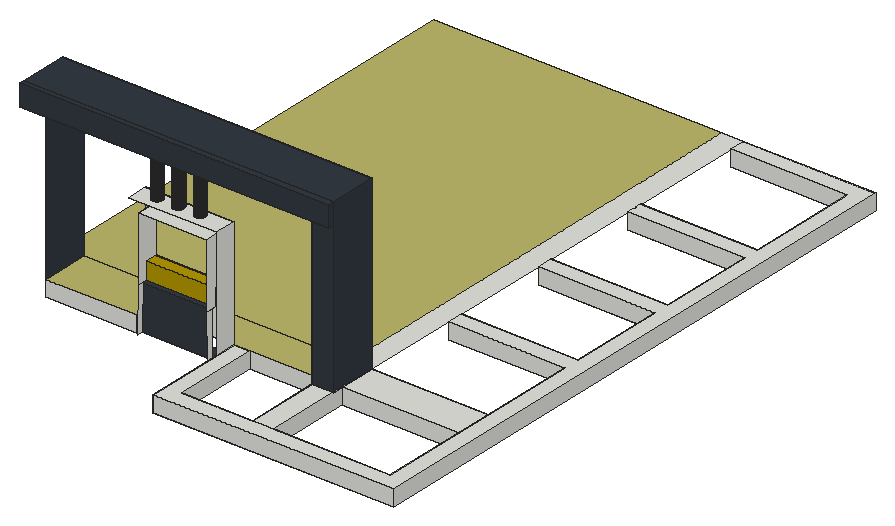
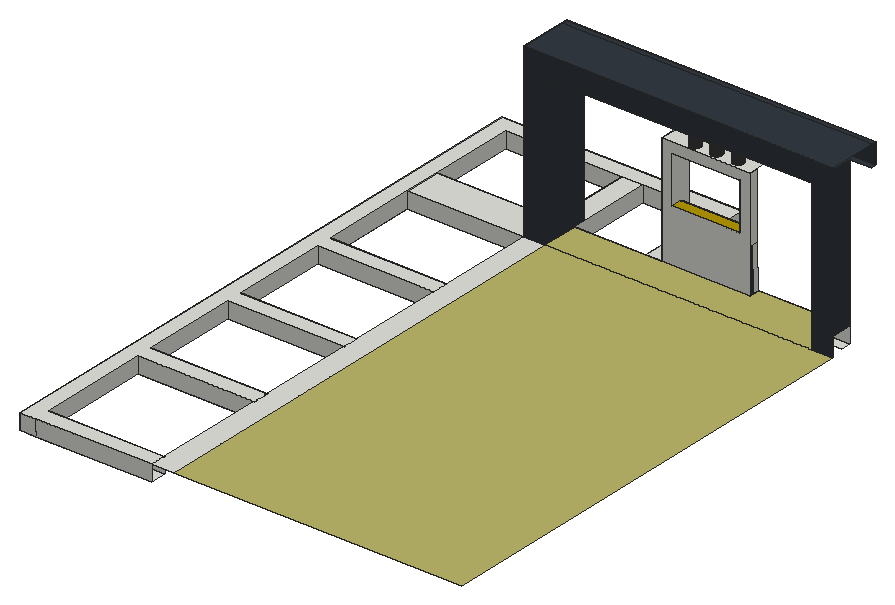
# SketchUp Ruby script. Lengths in inches.
U = 1.inch
M = Sketchup.active_model
def pt(a) = Geom::Point3d.new(a.map { |v| v * U })
def face(e, loops, mat)
  f = e.add_face(loops[0].map { |a| pt(a) })
  loops[1..].each { |l| e.add_face(l.map { |a| pt(a) }).erase! }
  f.material = f.back_material = mat if mat
  f
end
# faces: each face lists its corners as indices into pts; further lists are holes
def faces(e, pts, list, mat = nil) = list.each { |f| face(e, (f[0].is_a?(Array) ? f : [f]).map { |l| l.map { |i| pts[i] } }, mat) }
# xy, xz, yz: faces in a plane at the given z, y or x. An outline is a flat list of corners, or four numbers for a rectangle; further outlines are holes
def ring(l) = l.size == 4 ? [[l[0], l[1]], [l[2], l[1]], [l[2], l[3]], [l[0], l[3]]] : l.each_slice(2).to_a
def flat(e, list, mat, &to3) = list.each { |f| face(e, (f[0].is_a?(Array) ? f : [f]).map { |l| ring(l).map { |u, v| to3.(u, v) } }, mat) }
def xy(e, z, list, mat = nil) = flat(e, list, mat) { |x, y| [x, y, z] }
def xz(e, y, list, mat = nil) = flat(e, list, mat) { |x, z| [x, y, z] }
def yz(e, x, list, mat = nil) = flat(e, list, mat) { |y, z| [x, y, z] }
def lines(e, pts, list) = list.each { |a, b| e.add_line(pt(pts[a]), pt(pts[b])) }
# prism: a flat outline (further loops are holes) pulled along v
def prism(e, loops, v, mat = nil)
  f = face(e, loops, mat); d = Geom::Vector3d.new(v.map { |x| x * U })
  f.pushpull(f.normal.samedirection?(d) ? d.length : -d.length)
end
def box(e, o, s, mat = nil) = prism(e, [[o, [o[0] + s[0], o[1], o[2]], [o[0] + s[0], o[1] + s[1], o[2]], [o[0], o[1] + s[1], o[2]]]], [0, 0, s[2]], mat)
def at(x, y, z, deg = 0) = Geom::Transformation.translation(pt([x, y, z])) * Geom::Transformation.rotation(ORIGIN, Z_AXIS, deg.degrees)
def axes(o, x, y, z) = Geom::Transformation.new([*x, 0, *y, 0, *z, 0, *pt(o).to_a, 1])
def part(name) = M.definitions.add(name)
# library, detail: a bought-in or finely detailed component or shape, given as its bounding box
def library(name, o, s) = part(name).tap { |d| box(d.entities, o, s) }
def detail(e, o, s) = box(e.add_group.entities, o, s)
def put(e, d, t, mat = nil) = e.add_instance(d, t).tap { |i| i.material = mat if mat }
def group(e, t, mat = nil) = e.add_group.tap { |g| g.transformation = t; g.material = mat if mat }.entities
root = M.entities
M.materials.add("[0046_Gold]").color = [178, 150, 0]
M.materials.add("[0057_DarkKhaki]").color = [188, 182, 106]
M.materials.add("[0111_SlateGray]").color = [51, 58, 66]
xy(root,810,[[388.78,0,388.78,114,406.78,114,406.78,18,486,18,486,114,510,114,510,18,641,18,641,264,510,264,510,282,641,282,641,390,510,390,510,408,641,408,641,516,510,516,510,534,641,534,641,678,659,678,659,0],[186,102,288.84,114],[510,114,641,156],[510,660,641,678]])
xy(root,817.66,[[299.18,96,378.44,114]],"[0111_SlateGray]")
xy(root,828,[[388.78,0,659,0,659,678,510,678,510,660,641,660,641,534,510,534,510,516,641,516,641,408,510,408,510,390,641,390,641,282,510,282,510,264,641,264,641,18,406.78,18,406.78,114,388.78,114],[486,18,510,102],[486,102,510,114],[486,114,510,156],[510,114,641,156],
  [486,156,510,678]])
xy(root,828,[[186,102,288.84,102,288.84,114,486,114,486,156,186,156],[162,156,486,678]],"[0057_DarkKhaki]")
xy(root,867.66,[[300.19,96,377.43,101]],"[0111_SlateGray]")
xy(root,887.35,[[300.19,101,377.43,114]],"[0046_Gold]")
xy(root,940.57,[[300.19,90,377.43,114]])
xy(root,951.92,[[[288.84,90,388.78,114],[309.5,98.9375,308.875,98.96,308.25,99.05,307.64,99.21,307.05,99.43,306.49,99.71,305.96,100.04,305.47,100.43,305.02,100.87,304.62,101.35,304.27,101.875,303.98,102.43,303.74,103.01,303.58,103.62,303.47,104.24,303.43,104.87,303.45,105.49,303.55,106.11,303.7,106.72,303.92,107.3125,304.2,107.875,304.53,108.41,304.92,108.9,305.36,109.35,305.84,109.75,306.37,110.1,306.92,110.39,307.51,110.62,308.11,110.79,308.73,110.9,309.36,110.9375,309.98,110.91,310.61,110.82,311.21,110.67,311.8,110.45,312.37,110.17,312.9,109.83,313.39,109.44,313.84,109.01,314.24,108.52,314.59,108,314.88,107.44,315.11,106.86,315.28,106.26,315.39,105.64,315.43,105.01,315.4,104.38,315.3125,103.76,315.16,103.15,314.9375,102.5625,314.66,102,314.32,101.47,313.94,100.98,313.5,100.53,313.01,100.125,312.49,99.78,311.93,99.49,311.35,99.25,310.75,99.08,310.13,98.98],[333.5,99.0625,332.875,99.09,332.25,99.18,331.64,99.33,331.05,99.55,330.49,99.83,329.96,100.17,329.47,100.56,329.02,100.99,328.62,101.48,328.27,102,327.98,102.56,327.74,103.14,327.58,103.74,327.47,104.36,327.43,104.99,327.45,105.62,327.55,106.24,327.7,106.85,327.92,107.4375,328.2,108,328.53,108.53,328.92,109.02,329.36,109.47,329.84,109.875,330.37,110.22,330.92,110.51,331.51,110.75,332.11,110.92,332.73,111.02,333.36,111.0625,333.98,111.04,334.61,110.95,335.21,110.79,335.8,110.57,336.37,110.29,336.9,109.96,337.39,109.57,337.84,109.13,338.24,108.65,338.59,108.125,338.88,107.57,339.11,106.99,339.28,106.38,339.39,105.76,339.43,105.13,339.4,104.51,339.3125,103.89,339.16,103.28,338.9375,102.6875,338.66,102.125,338.32,101.59,337.94,101.1,337.5,100.65,337.01,100.25,336.49,99.9,335.93,99.61,335.35,99.38,334.75,99.21,334.13,99.1],[357.5,99.625,356.875,99.65,356.25,99.74,355.64,99.9,355.05,100.11,354.49,100.39,353.96,100.73,353.47,101.12,353.02,101.56,352.62,102.04,352.27,102.5625,351.98,103.12,351.74,103.7,351.58,104.31,351.47,104.93,351.43,105.55,351.45,106.18,351.55,106.8,351.7,107.41,351.92,108,352.2,108.5625,352.53,109.09,352.92,109.59,353.36,110.04,353.84,110.4375,354.37,110.78,354.92,111.08,355.51,111.31,356.11,111.48,356.73,111.58,357.36,111.625,357.98,111.6,358.61,111.51,359.21,111.35,359.8,111.14,360.37,110.86,360.9,110.52,361.39,110.13,361.84,109.69,362.24,109.21,362.59,108.6875,362.88,108.13,363.11,107.55,363.28,106.94,363.39,106.32,363.43,105.7,363.4,105.07,363.3125,104.45,363.16,103.84,362.9375,103.25,362.66,102.6875,362.32,102.16,361.94,101.66,361.5,101.21,361.01,100.8125,360.49,100.47,359.93,100.17,359.35,99.94,358.75,99.77,358.13,99.67]],[309.5,98.9375,308.875,98.96,308.25,99.05,307.64,99.21,307.05,99.43,306.49,99.71,305.96,100.04,305.47,100.43,305.02,100.87,304.62,101.35,304.27,101.875,303.98,102.43,303.74,103.01,303.58,103.62,303.47,104.24,303.43,104.87,303.45,105.49,303.55,106.11,303.7,106.72,303.92,107.3125,304.2,107.875,304.53,108.41,304.92,108.9,305.36,109.35,305.84,109.75,306.37,110.1,306.92,110.39,307.51,110.62,308.11,110.79,308.73,110.9,309.36,110.9375,309.98,110.91,310.61,110.82,311.21,110.67,311.8,110.45,312.37,110.17,312.9,109.83,313.39,109.44,313.84,109.01,314.24,108.52,314.59,108,314.88,107.44,315.11,106.86,315.28,106.26,315.39,105.64,315.43,105.01,315.4,104.38,315.3125,103.76,315.16,103.15,314.9375,102.5625,314.66,102,314.32,101.47,313.94,100.98,313.5,100.53,313.01,100.125,312.49,99.78,311.93,99.49,311.35,99.25,310.75,99.08,310.13,98.98],[333.5,99.0625,332.875,99.09,332.25,99.18,331.64,99.33,331.05,99.55,330.49,99.83,329.96,100.17,329.47,100.56,329.02,100.99,328.62,101.48,328.27,102,327.98,102.56,327.74,103.14,327.58,103.74,327.47,104.36,327.43,104.99,327.45,105.62,327.55,106.24,327.7,106.85,327.92,107.4375,328.2,108,328.53,108.53,328.92,109.02,329.36,109.47,329.84,109.875,330.37,110.22,330.92,110.51,331.51,110.75,332.11,110.92,332.73,111.02,333.36,111.0625,333.98,111.04,334.61,110.95,335.21,110.79,335.8,110.57,336.37,110.29,336.9,109.96,337.39,109.57,337.84,109.13,338.24,108.65,338.59,108.125,338.88,107.57,339.11,106.99,339.28,106.38,339.39,105.76,339.43,105.13,339.4,104.51,339.3125,103.89,339.16,103.28,338.9375,102.6875,338.66,102.125,338.32,101.59,337.94,101.1,337.5,100.65,337.01,100.25,336.49,99.9,335.93,99.61,335.35,99.38,334.75,99.21,334.13,99.1],[357.5,99.625,356.875,99.65,356.25,99.74,355.64,99.9,355.05,100.11,354.49,100.39,353.96,100.73,353.47,101.12,353.02,101.56,352.62,102.04,352.27,102.5625,351.98,103.12,351.74,103.7,351.58,104.31,351.47,104.93,351.43,105.55,351.45,106.18,351.55,106.8,351.7,107.41,351.92,108,352.2,108.5625,352.53,109.09,352.92,109.59,353.36,110.04,353.84,110.4375,354.37,110.78,354.92,111.08,355.51,111.31,356.11,111.48,356.73,111.58,357.36,111.625,357.98,111.6,358.61,111.51,359.21,111.35,359.8,111.14,360.37,110.86,360.9,110.52,361.39,110.13,361.84,109.69,362.24,109.21,362.59,108.6875,362.88,108.13,363.11,107.55,363.28,106.94,363.39,106.32,363.43,105.7,363.4,105.07,363.3125,104.45,363.16,103.84,362.9375,103.25,362.66,102.6875,362.32,102.16,361.94,101.66,361.5,101.21,361.01,100.8125,360.49,100.47,359.93,100.17,359.35,99.94,358.75,99.77,358.13,99.67]])
xy(root,996,[[309.5,98.9375,310.13,98.98,310.75,99.08,311.35,99.25,311.93,99.49,312.49,99.78,313.01,100.125,313.5,100.53,313.94,100.98,314.32,101.47,314.66,102,304.2,102,304.27,101.875,304.62,101.35,305.02,100.87,305.47,100.43,305.96,100.04,306.49,99.71,307.05,99.43,307.64,99.21,308.25,99.05,308.875,98.96],[333.5,99.0625,334.13,99.1,334.75,99.21,335.35,99.38,335.93,99.61,336.49,99.9,337.01,100.25,337.5,100.65,337.94,101.1,338.32,101.59,338.58,102,328.27,102,328.62,101.48,329.02,100.99,329.47,100.56,329.96,100.17,330.49,99.83,331.05,99.55,331.64,99.33,332.25,99.18,332.875,99.09],[357.5,99.625,358.13,99.67,358.75,99.77,359.35,99.94,359.93,100.17,360.49,100.47,361.01,100.8125,361.5,101.21,361.94,101.66,362.2,102,352.65,102,353.02,101.56,353.47,101.12,353.96,100.73,354.49,100.39,355.05,100.11,355.64,99.9,356.25,99.74,356.875,99.65],[304.2,102,314.66,102,314.9375,102.5625,315.16,103.15,315.3125,103.76,315.4,104.38,315.43,105.01,315.39,105.64,315.28,106.26,315.11,106.86,314.88,107.44,314.59,108,314.24,108.52,313.84,109.01,313.39,109.44,312.9,109.83,312.37,110.17,311.8,110.45,311.21,110.67,310.61,110.82,309.98,110.91,309.36,110.9375,308.73,110.9,308.11,110.79,307.51,110.62,306.92,110.39,306.37,110.1,305.84,109.75,305.36,109.35,304.92,108.9,304.53,108.41,304.2,107.875,303.92,107.3125,303.7,106.72,303.55,106.11,303.45,105.49,303.43,104.87,303.47,104.24,303.58,103.62,303.74,103.01,303.98,102.43],[328.27,102,338.58,102,338.66,102.125,338.9375,102.6875,339.16,103.28,339.3125,103.89,339.4,104.51,339.43,105.13,339.39,105.76,339.28,106.38,339.11,106.99,338.88,107.57,338.59,108.125,338.24,108.65,337.84,109.13,337.39,109.57,336.9,109.96,336.37,110.29,335.8,110.57,335.21,110.79,334.61,110.95,333.98,111.04,333.36,111.0625,332.73,111.02,332.11,110.92,331.51,110.75,330.92,110.51,330.37,110.22,329.84,109.875,329.36,109.47,328.92,109.02,328.53,108.53,328.2,108,327.92,107.4375,327.7,106.85,327.55,106.24,327.45,105.62,327.43,104.99,327.47,104.36,327.58,103.74,327.74,103.14,327.98,102.56],
  [352.65,102,362.2,102,362.32,102.16,362.66,102.6875,362.9375,103.25,363.16,103.84,363.3125,104.45,363.4,105.07,363.43,105.7,363.39,106.32,363.28,106.94,363.11,107.55,362.88,108.13,362.59,108.6875,362.24,109.21,361.84,109.69,361.39,110.13,360.9,110.52,360.37,110.86,359.8,111.14,359.21,111.35,358.61,111.51,357.98,111.6,357.36,111.625,356.73,111.58,356.11,111.48,355.51,111.31,354.92,111.08,354.37,110.78,353.84,110.4375,353.36,110.04,352.92,109.59,352.53,109.09,352.2,108.5625,351.92,108,351.7,107.41,351.55,106.8,351.45,106.18,351.43,105.55,351.47,104.93,351.58,104.31,351.74,103.7,351.98,103.12,352.27,102.5625,352.62,102.04],[239.33,115.14,238.07,115.2,236.83,115.39,235.61,115.71,234.4375,116.15,233.32,116.71,232.26,117.39,231.28,118.17,230.38,119.06,229.59,120.03,228.9,121.08,228.32,122.19,227.86,123.36,227.53,124.57,227.32,125.8125,227.25,127.07,227.31,128.32,227.5,129.5625,227.8125,130.78,228.26,131.95,228.82,133.08,229.5,134.13,230.28,135.12,231.16,136.01,232.13,136.81,233.18,137.5,234.3,138.07,235.47,138.53,236.68,138.87,237.92,139.07,239.17,139.14,240.43,139.09,241.67,138.9,242.88,138.58,244.06,138.14,245.18,137.57,246.24,136.9,247.22,136.11,248.11,135.23,248.91,134.26,249.6,133.21,250.18,132.09,250.64,130.93,250.97,129.71,251.17,128.47,251.25,127.22,251.19,125.97,251,124.72,250.69,123.51,250.24,122.33,249.68,121.21,249,120.15,248.22,119.17,247.34,118.28,246.36,117.48,245.32,116.79,244.2,116.21,243.03,115.76,241.82,115.42,240.58,115.22],[442.51,115.14,441.26,115.2,440.02,115.39,438.8,115.71,437.625,116.15,436.5,116.71,435.45,117.39,434.46,118.17,433.57,119.06,432.77,120.03,432.08,121.08,431.51,122.19,431.05,123.36,430.72,124.57,430.51,125.8125,430.4375,127.07,430.49,128.32,430.68,129.5625,431,130.78,431.44,131.95,432.01,133.08,432.68,134.13,433.47,135.12,434.35,136.01,435.32,136.81,436.37,137.5,437.49,138.07,438.65,138.53,439.87,138.87,441.11,139.07,442.36,139.14,443.61,139.09,444.86,138.9,446.07,138.58,447.25,138.14,448.37,137.57,449.43,136.9,450.41,136.11,451.3,135.23,452.1,134.26,452.79,133.21,453.37,132.09,453.83,130.93,454.16,129.71,454.36,128.47,454.4375,127.22,454.38,125.97,454.19,124.72,453.87,123.51,453.43,122.33,452.87,121.21,452.19,120.15,451.41,119.17,450.52,118.28,449.55,117.48,448.5,116.79,447.39,116.21,446.22,115.76,445.01,115.42,443.77,115.22]])
xy(root,996,[[[162,96,162,102,186,102,186,156,486,156,486,102,510,102,510,96],[442.51,115.14,443.77,115.22,445.01,115.42,446.22,115.76,447.39,116.21,448.5,116.79,449.55,117.48,450.52,118.28,451.41,119.17,452.19,120.15,452.87,121.21,453.43,122.33,453.87,123.51,454.19,124.72,454.38,125.97,454.4375,127.22,454.36,128.47,454.16,129.71,453.83,130.93,453.37,132.09,452.79,133.21,452.1,134.26,451.3,135.23,450.41,136.11,449.43,136.9,448.37,137.57,447.25,138.14,446.07,138.58,444.86,138.9,443.61,139.09,442.36,139.14,441.11,139.07,439.87,138.87,438.65,138.53,437.49,138.07,436.37,137.5,435.32,136.81,434.35,136.01,433.47,135.12,432.68,134.13,432.01,133.08,431.44,131.95,431,130.78,430.68,129.5625,430.49,128.32,430.4375,127.07,430.51,125.8125,430.72,124.57,431.05,123.36,431.51,122.19,432.08,121.08,432.77,120.03,433.57,119.06,434.46,118.17,435.45,117.39,436.5,116.71,437.625,116.15,438.8,115.71,440.02,115.39,441.26,115.2],[239.33,115.14,240.58,115.22,241.82,115.42,243.03,115.76,244.2,116.21,245.32,116.79,246.36,117.48,247.34,118.28,248.22,119.17,249,120.15,249.68,121.21,250.24,122.33,250.69,123.51,251,124.72,251.19,125.97,251.25,127.22,251.17,128.47,250.97,129.71,250.64,130.93,250.18,132.09,249.6,133.21,248.91,134.26,248.11,135.23,247.22,136.11,246.24,136.9,245.18,137.57,244.06,138.14,242.88,138.58,241.67,138.9,240.43,139.09,239.17,139.14,237.92,139.07,236.68,138.87,235.47,138.53,234.3,138.07,233.18,137.5,232.13,136.81,231.16,136.01,230.28,135.12,229.5,134.13,228.82,133.08,228.26,131.95,227.8125,130.78,227.5,129.5625,227.31,128.32,227.25,127.07,227.32,125.8125,227.53,124.57,227.86,123.36,228.32,122.19,228.9,121.08,229.59,120.03,230.38,119.06,231.28,118.17,232.26,117.39,233.32,116.71,234.4375,116.15,235.61,115.71,236.83,115.39,238.07,115.2],[357.5,99.625,358.13,99.67,358.75,99.77,359.35,99.94,359.93,100.17,360.49,100.47,361.01,100.8125,361.5,101.21,361.94,101.66,362.2,102,362.32,102.16,362.66,102.6875,362.9375,103.25,363.16,103.84,363.3125,104.45,363.4,105.07,363.43,105.7,363.39,106.32,363.28,106.94,363.11,107.55,362.88,108.13,362.59,108.6875,362.24,109.21,361.84,109.69,361.39,110.13,360.9,110.52,360.37,110.86,359.8,111.14,359.21,111.35,358.61,111.51,357.98,111.6,357.36,111.625,356.73,111.58,356.11,111.48,355.51,111.31,354.92,111.08,354.37,110.78,353.84,110.4375,353.36,110.04,352.92,109.59,352.53,109.09,352.2,108.5625,351.92,108,351.7,107.41,351.55,106.8,351.45,106.18,351.43,105.55,351.47,104.93,351.58,104.31,351.74,103.7,351.98,103.12,352.27,102.5625,352.62,102.04,352.65,102,353.02,101.56,353.47,101.12,353.96,100.73,354.49,100.39,355.05,100.11,355.64,99.9,356.25,99.74,356.875,99.65],[333.5,99.0625,334.13,99.1,334.75,99.21,335.35,99.38,335.93,99.61,336.49,99.9,337.01,100.25,337.5,100.65,337.94,101.1,338.32,101.59,338.58,102,338.66,102.125,338.9375,102.6875,339.16,103.28,339.3125,103.89,339.4,104.51,339.43,105.13,339.39,105.76,339.28,106.38,339.11,106.99,338.88,107.57,338.59,108.125,338.24,108.65,337.84,109.13,337.39,109.57,336.9,109.96,336.37,110.29,335.8,110.57,335.21,110.79,334.61,110.95,333.98,111.04,333.36,111.0625,332.73,111.02,332.11,110.92,331.51,110.75,330.92,110.51,330.37,110.22,329.84,109.875,329.36,109.47,328.92,109.02,328.53,108.53,328.2,108,327.92,107.4375,327.7,106.85,327.55,106.24,327.45,105.62,327.43,104.99,327.47,104.36,327.58,103.74,327.74,103.14,327.98,102.56,328.27,102,328.62,101.48,329.02,100.99,329.47,100.56,329.96,100.17,330.49,99.83,331.05,99.55,331.64,99.33,332.25,99.18,332.875,99.09],[309.5,98.9375,310.13,98.98,310.75,99.08,311.35,99.25,311.93,99.49,312.49,99.78,313.01,100.125,313.5,100.53,313.94,100.98,314.32,101.47,314.66,102,314.9375,102.5625,315.16,103.15,315.3125,103.76,315.4,104.38,315.43,105.01,315.39,105.64,315.28,106.26,315.11,106.86,314.88,107.44,314.59,108,314.24,108.52,313.84,109.01,313.39,109.44,312.9,109.83,312.37,110.17,311.8,110.45,311.21,110.67,310.61,110.82,309.98,110.91,309.36,110.9375,308.73,110.9,308.11,110.79,307.51,110.62,306.92,110.39,306.37,110.1,305.84,109.75,305.36,109.35,304.92,108.9,304.53,108.41,304.2,107.875,303.92,107.3125,303.7,106.72,303.55,106.11,303.45,105.49,303.43,104.87,303.47,104.24,303.58,103.62,303.74,103.01,303.98,102.43,304.2,102,304.27,101.875,304.62,101.35,305.02,100.87,305.47,100.43,305.96,100.04,306.49,99.71,307.05,99.43,307.64,99.21,308.25,99.05,308.875,98.96]]],"[0111_SlateGray]")
xy(root,1020,[[162,96,510,102],[162,102,510,156]],"[0111_SlateGray]")
xz(root,0,[[388.78,810,659,828]])
xz(root,18,[[406.78,810,486,828],[510,810,641,828]])
xz(root,96,[[299.18,817.66,378.44,817.66,377.43,867.66,300.19,867.66],[162,996,510,1020]],"[0111_SlateGray]")
xz(root,101,[[300.19,867.66,377.43,887.35]],"[0046_Gold]")
xz(root,102,[[186,810,288.84,828]])
xz(root,102,[[486,828,510,996]],"[0111_SlateGray]")
xz(root,114,[[388.78,810,406.78,828],[406.78,810,486,828],[486,810,510,828],[510,810,641,828],[[288.84,828,388.78,951.92],[300.19,887.35,377.43,940.57]]])
xz(root,156,[[510,810,641,828]])
xz(root,156,[[162,828,162,1020,510,1020,510,828,486,828,486,996,186,996,186,828]],"[0111_SlateGray]")
xz(root,264,[[510,810,641,828]])
xz(root,282,[[510,810,641,828]])
xz(root,390,[[510,810,641,828]])
xz(root,408,[[510,810,641,828]])
xz(root,516,[[510,810,641,828]])
xz(root,534,[[510,810,641,828]])
xz(root,660,[[510,810,641,828]])
xz(root,678,[[510,810,641,828],[641,810,659,828]])
yz(root,186,[[102,828,156,996]],"[0111_SlateGray]")
yz(root,288.84,[[102,810,114,828]])
yz(root,300.19,[[90,867.66,101,867.66,101,887.35,114,887.35,114,940.57,90,940.57]])
yz(root,377.43,[[90,867.66,90,940.57,114,940.57,114,887.35,101,887.35,101,867.66]])
yz(root,388.78,[[0,810,90,828],[90,810,114,828],[90,828,114,951.92]])
yz(root,406.78,[[18,810,114,828]])
yz(root,486,[[18,810,114,828]])
yz(root,486,[[102,828,156,996]],"[0111_SlateGray]")
yz(root,510,[[18,810,114,828],[114,810,156,828]])
yz(root,510,[[102,828,156,1020],[96,996,102,1020]],"[0111_SlateGray]")
yz(root,641,[[18,810,114,828],[114,810,156,828],[156,810,264,828],[282,810,390,828],[408,810,516,828],
  [534,810,660,828]])
yz(root,659,[[0,810,678,828]])
p = [[300.19,90,867.66],[299.18,90,817.66],[299.18,96,817.66],[300.19,96,867.66],[378.44,90,817.66],[377.43,90,867.66],
  [377.43,96,867.66],[378.44,96,817.66],[308.875,98.96,951.92],[309.5,98.9375,951.92],[309.5,98.9375,996],[308.875,98.96,996],
  [310.13,98.98,951.92],[310.13,98.98,996],[308.25,99.05,951.92],[308.25,99.05,996],[310.75,99.08,951.92],[310.75,99.08,996],
  [307.64,99.21,951.92],[307.64,99.21,996],[311.35,99.25,951.92],[311.35,99.25,996],[332.25,99.18,951.92],[332.875,99.09,951.92],
  [332.875,99.09,996],[332.25,99.18,996],[333.5,99.0625,951.92],[333.5,99.0625,996],[334.13,99.1,951.92],[334.13,99.1,996],
  [334.75,99.21,951.92],[334.75,99.21,996],[307.05,99.43,951.92],[307.05,99.43,996],[331.64,99.33,951.92],[331.64,99.33,996],
  [335.35,99.38,951.92],[335.35,99.38,996],[311.93,99.49,951.92],[311.93,99.49,996],[331.05,99.55,951.92],[331.05,99.55,996],
  [306.49,99.71,951.92],[306.49,99.71,996],[335.93,99.61,951.92],[335.93,99.61,996],[312.49,99.78,951.92],[312.49,99.78,996],
  [330.49,99.83,951.92],[330.49,99.83,996],[336.49,99.9,951.92],[336.49,99.9,996],[356.875,99.65,951.92],[357.5,99.625,951.92],
  [357.5,99.625,996],[356.875,99.65,996],[358.13,99.67,951.92],[358.13,99.67,996],[305.96,100.04,951.92],[305.96,100.04,996],
  [355.64,99.9,951.92],[356.25,99.74,951.92],[356.25,99.74,996],[355.64,99.9,996],[358.75,99.77,951.92],[358.75,99.77,996],
  [313.01,100.125,951.92],[313.01,100.125,996],[329.96,100.17,951.92],[329.96,100.17,996],[359.35,99.94,951.92],[359.35,99.94,996],
  [337.01,100.25,951.92],[337.01,100.25,996],[355.05,100.11,951.92],[355.05,100.11,996],[359.93,100.17,951.92],[359.93,100.17,996],
  [305.47,100.43,951.92],[305.47,100.43,996],[313.5,100.53,951.92],[313.5,100.53,996],[354.49,100.39,951.92],[354.49,100.39,996],
  [329.47,100.56,951.92],[329.47,100.56,996],[360.49,100.47,951.92],[360.49,100.47,996],[337.5,100.65,951.92],[337.5,100.65,996],
  [305.02,100.87,951.92],[305.02,100.87,996],[353.96,100.73,951.92],[353.96,100.73,996],[313.94,100.98,951.92],[313.94,100.98,996],
  [361.01,100.8125,951.92],[361.01,100.8125,996],[329.02,100.99,951.92],[329.02,100.99,996],[337.94,101.1,951.92],[337.94,101.1,996],
  [353.47,101.12,951.92],[353.47,101.12,996],[361.5,101.21,951.92],[361.5,101.21,996],[304.62,101.35,951.92],[304.62,101.35,996],
  [314.32,101.47,951.92],[314.32,101.47,996],[328.62,101.48,951.92],[328.62,101.48,996],[338.32,101.59,951.92],[338.32,101.59,996],
  [353.02,101.56,951.92],[353.02,101.56,996],[361.94,101.66,951.92],[361.94,101.66,996],[304.27,101.875,951.92],[304.27,101.875,996],
  [314.66,102,951.92],[314.66,102,996],[328.27,102,951.92],[328.27,102,996],[338.66,102.125,951.92],[338.66,102.125,996],
  [338.58,102,996],[352.62,102.04,951.92],[352.65,102,996],[352.62,102.04,996],[362.32,102.16,951.92],[362.32,102.16,996],
  [362.2,102,996],[303.98,102.43,951.92],[304.2,102,996],[303.98,102.43,996],[314.9375,102.5625,951.92],[314.9375,102.5625,996],
  [327.98,102.56,951.92],[327.98,102.56,996],[352.27,102.5625,951.92],[352.27,102.5625,996],[338.9375,102.6875,951.92],[338.9375,102.6875,996],
  [362.66,102.6875,951.92],[362.66,102.6875,996],[303.74,103.01,951.92],[303.74,103.01,996],[315.16,103.15,951.92],[315.16,103.15,996],
  [327.74,103.14,951.92],[327.74,103.14,996],[351.98,103.12,951.92],[351.98,103.12,996],[339.16,103.28,951.92],[339.16,103.28,996],
  [362.9375,103.25,951.92],[362.9375,103.25,996],[303.58,103.62,951.92],[303.58,103.62,996],[327.58,103.74,951.92],[327.58,103.74,996],
  [351.74,103.7,951.92],[351.74,103.7,996],[315.3125,103.76,951.92],[315.3125,103.76,996],[339.3125,103.89,951.92],[339.3125,103.89,996],
  [363.16,103.84,951.92],[363.16,103.84,996],[303.47,104.24,951.92],[303.47,104.24,996],[327.47,104.36,951.92],[327.47,104.36,996],
  [351.58,104.31,951.92],[351.58,104.31,996],[315.4,104.38,951.92],[315.4,104.38,996],[363.3125,104.45,951.92],[363.3125,104.45,996],
  [339.4,104.51,951.92],[339.4,104.51,996],[303.43,104.87,951.92],[303.43,104.87,996],[351.47,104.93,951.92],[351.47,104.93,996],
  [315.43,105.01,951.92],[315.43,105.01,996],[327.43,104.99,951.92],[327.43,104.99,996],[363.4,105.07,951.92],[363.4,105.07,996],
  [339.43,105.13,951.92],[339.43,105.13,996],[303.45,105.49,951.92],[303.45,105.49,996],[351.43,105.55,951.92],[351.43,105.55,996],
  [315.39,105.64,951.92],[315.39,105.64,996],[327.45,105.62,951.92],[327.45,105.62,996],[339.39,105.76,951.92],[339.39,105.76,996],
  [363.43,105.7,951.92],[363.43,105.7,996],[303.55,106.11,951.92],[303.55,106.11,996],[315.28,106.26,951.92],[315.28,106.26,996],
  [327.55,106.24,951.92],[327.55,106.24,996],[351.45,106.18,951.92],[351.45,106.18,996],[363.39,106.32,951.92],[363.39,106.32,996],
  [339.28,106.38,951.92],[339.28,106.38,996],[303.7,106.72,951.92],[303.7,106.72,996],[327.7,106.85,951.92],[327.7,106.85,996],
  [351.55,106.8,951.92],[351.55,106.8,996],[315.11,106.86,951.92],[315.11,106.86,996],[363.28,106.94,951.92],[363.28,106.94,996],
  [339.11,106.99,951.92],[339.11,106.99,996],[303.92,107.3125,951.92],[303.92,107.3125,996],[327.92,107.4375,951.92],[327.92,107.4375,996],
  [351.7,107.41,951.92],[351.7,107.41,996],[314.88,107.44,951.92],[314.88,107.44,996],[363.11,107.55,951.92],[363.11,107.55,996],
  [338.88,107.57,951.92],[338.88,107.57,996],[304.2,107.875,951.92],[304.2,107.875,996],[314.59,108,951.92],[314.59,108,996],
  [328.2,108,951.92],[328.2,108,996],[351.92,108,951.92],[351.92,108,996],[362.88,108.13,951.92],[362.88,108.13,996],
  [338.59,108.125,951.92],[338.59,108.125,996],[304.53,108.41,951.92],[304.53,108.41,996],[314.24,108.52,951.92],[314.24,108.52,996],
  [328.53,108.53,951.92],[328.53,108.53,996],[352.2,108.5625,951.92],[352.2,108.5625,996],[338.24,108.65,951.92],[338.24,108.65,996],
  [362.59,108.6875,951.92],[362.59,108.6875,996],[304.92,108.9,951.92],[304.92,108.9,996],[313.84,109.01,951.92],[313.84,109.01,996],
  [328.92,109.02,951.92],[328.92,109.02,996],[337.84,109.13,951.92],[337.84,109.13,996],[352.53,109.09,951.92],[352.53,109.09,996],
  [362.24,109.21,951.92],[362.24,109.21,996],[305.36,109.35,951.92],[305.36,109.35,996],[313.39,109.44,951.92],[313.39,109.44,996],
  [329.36,109.47,951.92],[329.36,109.47,996],[337.39,109.57,951.92],[337.39,109.57,996],[352.92,109.59,951.92],[352.92,109.59,996],
  [361.84,109.69,951.92],[361.84,109.69,996],[305.84,109.75,951.92],[305.84,109.75,996],[312.9,109.83,951.92],[312.9,109.83,996],
  [329.84,109.875,951.92],[329.84,109.875,996],[336.9,109.96,951.92],[336.9,109.96,996],[353.36,110.04,951.92],[353.36,110.04,996],
  [306.37,110.1,951.92],[306.37,110.1,996],[361.39,110.13,951.92],[361.39,110.13,996],[312.37,110.17,951.92],[312.37,110.17,996],
  [330.37,110.22,951.92],[330.37,110.22,996],[336.37,110.29,951.92],[336.37,110.29,996],[353.84,110.4375,951.92],[353.84,110.4375,996],
  [306.92,110.39,951.92],[306.92,110.39,996],[360.9,110.52,951.92],[360.9,110.52,996],[311.8,110.45,951.92],[311.8,110.45,996],
  [330.92,110.51,951.92],[330.92,110.51,996],[335.8,110.57,951.92],[335.8,110.57,996],[307.51,110.62,951.92],[307.51,110.62,996],
  [311.21,110.67,951.92],[311.21,110.67,996],[354.37,110.78,951.92],[354.37,110.78,996],[331.51,110.75,951.92],[331.51,110.75,996],
  [360.37,110.86,951.92],[360.37,110.86,996],[308.11,110.79,951.92],[308.11,110.79,996],[335.21,110.79,951.92],[335.21,110.79,996],
  [310.61,110.82,951.92],[310.61,110.82,996],[332.11,110.92,951.92],[332.11,110.92,996],[308.73,110.9,951.92],[308.73,110.9,996],
  [309.98,110.91,951.92],[309.98,110.91,996],[334.61,110.95,951.92],[334.61,110.95,996],[354.92,111.08,951.92],[354.92,111.08,996],
  [309.36,110.9375,951.92],[309.36,110.9375,996],[332.73,111.02,951.92],[332.73,111.02,996],[333.98,111.04,951.92],[333.98,111.04,996],
  [359.8,111.14,951.92],[359.8,111.14,996],[333.36,111.0625,951.92],[333.36,111.0625,996],[355.51,111.31,951.92],[355.51,111.31,996],
  [359.21,111.35,951.92],[359.21,111.35,996],[356.11,111.48,951.92],[356.11,111.48,996],[358.61,111.51,951.92],[358.61,111.51,996],
  [356.73,111.58,951.92],[356.73,111.58,996],[357.98,111.6,951.92],[357.98,111.6,996],[357.36,111.625,951.92],[357.36,111.625,996]]
faces(root,p,[[0,1,2,3],[4,5,6,7],[8,9,10,11],[9,12,13,10],[14,8,11,15],[12,16,17,13],[18,14,15,19],[16,20,21,17],
  [22,23,24,25],[23,26,27,24],[26,28,29,27],[28,30,31,29],[32,18,19,33],[34,22,25,35],[30,36,37,31],[20,38,39,21],
  [40,34,35,41],[42,32,33,43],[36,44,45,37],[38,46,47,39],[48,40,41,49],[44,50,51,45],[52,53,54,55],[53,56,57,54],
  [58,42,43,59],[60,61,62,63],[61,52,55,62],[56,64,65,57],[46,66,67,47],[68,48,49,69],[64,70,71,65],[50,72,73,51],
  [74,60,63,75],[70,76,77,71],[78,58,59,79],[66,80,81,67],[82,74,75,83],[84,68,69,85],[76,86,87,77],[72,88,89,73],
  [90,78,79,91],[92,82,83,93],[80,94,95,81],[86,96,97,87],[98,84,85,99],[88,100,101,89],[102,92,93,103],[96,104,105,97],
  [106,90,91,107],[94,108,109,95],[110,98,99,111],[100,112,113,101],[114,102,103,115],[104,116,117,105],[118,106,107,119],[108,120,121,109],
  [122,110,111,123],[112,124,125,126,113],[127,114,115,128,129],[116,130,131,132,117],[133,118,119,134,135],[120,136,137,121],[138,122,123,139],[140,127,129,141],
  [124,142,143,125],[130,144,145,131],[146,133,135,147],[136,148,149,137],[150,138,139,151],[152,140,141,153],[142,154,155,143],[144,156,157,145],
  [158,146,147,159],[160,150,151,161],[162,152,153,163],[148,164,165,149],[154,166,167,155],[156,168,169,157],[170,158,159,171],[172,160,161,173],
  [174,162,163,175],[164,176,177,165],[168,178,179,169],[166,180,181,167],[182,170,171,183],[184,174,175,185],[176,186,187,177],[188,172,173,189],
  [178,190,191,179],[180,192,193,181],[194,182,183,195],[196,184,185,197],[186,198,199,187],[200,188,189,201],[192,202,203,193],[190,204,205,191],
  [206,194,195,207],[198,208,209,199],[210,200,201,211],[212,196,197,213],[204,214,215,205],[202,216,217,203],[218,206,207,219],[220,210,211,221],
  [222,212,213,223],[208,224,225,209],[214,226,227,215],[216,228,229,217],[230,218,219,231],[232,220,221,233],[234,222,223,235],[224,236,237,225],
  [226,238,239,227],[228,240,241,229],[242,230,231,243],[236,244,245,237],[246,232,233,247],[248,234,235,249],[238,250,251,239],[240,252,253,241],
  [254,242,243,255],[244,256,257,245],[258,246,247,259],[260,248,249,261],[252,262,263,253],[250,264,265,251],[266,254,255,267],[256,268,269,257],
  [270,258,259,271],[262,272,273,263],[274,260,261,275],[264,276,277,265],[278,266,267,279],[268,280,281,269],[282,270,271,283],[272,284,285,273],
  [286,274,275,287],[276,288,289,277],[290,278,279,291],[280,292,293,281],[294,282,283,295],[284,296,297,285],[298,286,287,299],[300,290,291,301],
  [288,302,303,289],[292,304,305,293],[306,294,295,307],[296,308,309,297],[310,298,299,311],[312,300,301,313],[302,314,315,303],[304,316,317,305],
  [318,306,307,319],[308,320,321,309],[322,312,313,323],[316,324,325,317],[326,310,311,327],[328,318,319,329],[314,330,331,315],[332,322,323,333],
  [320,334,335,321],[324,336,337,325],[338,328,329,339],[340,332,333,341],[336,342,343,337],[334,344,345,335],[346,326,327,347],[348,340,341,349],
  [342,348,349,343],[350,338,339,351],[344,352,353,345],[330,354,355,331],[356,350,351,357],[352,356,357,353],[358,346,347,359],[354,360,361,355],
  [362,358,359,363],[360,364,365,361],[366,362,363,367],[364,368,369,365],[370,366,367,371],[368,370,371,369]])
